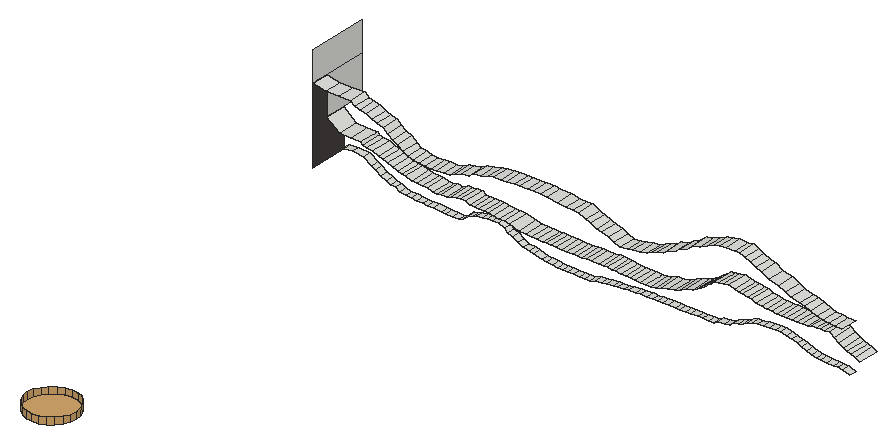
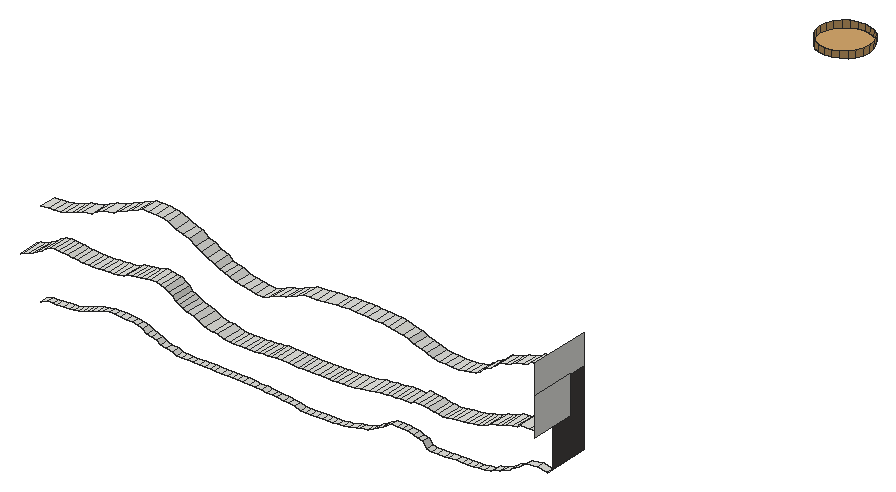
# SketchUp Ruby script. Lengths in inches.
U = 1.inch
M = Sketchup.active_model
def pt(a) = Geom::Point3d.new(a.map { |v| v * U })
def face(e, loops, mat)
  f = e.add_face(loops[0].map { |a| pt(a) })
  loops[1..].each { |l| e.add_face(l.map { |a| pt(a) }).erase! }
  f.material = f.back_material = mat if mat
  f
end
# faces: each face lists its corners as indices into pts; further lists are holes
def faces(e, pts, list, mat = nil) = list.each { |f| face(e, (f[0].is_a?(Array) ? f : [f]).map { |l| l.map { |i| pts[i] } }, mat) }
# xy, xz, yz: faces in a plane at the given z, y or x. An outline is a flat list of corners, or four numbers for a rectangle; further outlines are holes
def ring(l) = l.size == 4 ? [[l[0], l[1]], [l[2], l[1]], [l[2], l[3]], [l[0], l[3]]] : l.each_slice(2).to_a
def flat(e, list, mat, &to3) = list.each { |f| face(e, (f[0].is_a?(Array) ? f : [f]).map { |l| ring(l).map { |u, v| to3.(u, v) } }, mat) }
def xy(e, z, list, mat = nil) = flat(e, list, mat) { |x, y| [x, y, z] }
def xz(e, y, list, mat = nil) = flat(e, list, mat) { |x, z| [x, y, z] }
def yz(e, x, list, mat = nil) = flat(e, list, mat) { |y, z| [x, y, z] }
def lines(e, pts, list) = list.each { |a, b| e.add_line(pt(pts[a]), pt(pts[b])) }
# prism: a flat outline (further loops are holes) pulled along v
def prism(e, loops, v, mat = nil)
  f = face(e, loops, mat); d = Geom::Vector3d.new(v.map { |x| x * U })
  f.pushpull(f.normal.samedirection?(d) ? d.length : -d.length)
end
def box(e, o, s, mat = nil) = prism(e, [[o, [o[0] + s[0], o[1], o[2]], [o[0] + s[0], o[1] + s[1], o[2]], [o[0], o[1] + s[1], o[2]]]], [0, 0, s[2]], mat)
def at(x, y, z, deg = 0) = Geom::Transformation.translation(pt([x, y, z])) * Geom::Transformation.rotation(ORIGIN, Z_AXIS, deg.degrees)
def axes(o, x, y, z) = Geom::Transformation.new([*x, 0, *y, 0, *z, 0, *pt(o).to_a, 1])
def part(name) = M.definitions.add(name)
# library, detail: a bought-in or finely detailed component or shape, given as its bounding box
def library(name, o, s) = part(name).tap { |d| box(d.entities, o, s) }
def detail(e, o, s) = box(e.add_group.entities, o, s)
def put(e, d, t, mat = nil) = e.add_instance(d, t).tap { |i| i.material = mat if mat }
def group(e, t, mat = nil) = e.add_group.tap { |g| g.transformation = t; g.material = mat if mat }.entities
root = M.entities
M.materials.add("[Field Square Tile]").color = [211, 167, 108]
M.materials.add("[Granite Tile]1").color = [68, 65, 63]
xy(root,237.65,[[1160.83,2401.37,1161.52,2402.3],[1161.52,2401.37,1162.14,2402.3]])
xy(root,238.33,[[1169.93,2401.37,1170.48,2402.3],[1170.48,2401.37,1171.16,2402.3]])
xy(root,238.34,[[1171.84,2401.37,1172.77,2402.3],[1172.77,2401.37,1173.26,2402.3],[1173.26,2401.37,1174.02,2402.3],[1174.02,2401.37,1174.65,2402.3],[1174.65,2401.37,1175.4,2402.3],
  [1175.4,2401.37,1176.02,2402.3],[1176.02,2401.37,1176.79,2402.3],[1176.79,2401.37,1177.41,2402.3]])
xy(root,241.52,[[1131.53,2396.68,1131.59,2402.3]])
xy(root,241.68,[[1162.03,2398.8,1162.62,2401.37]])
xy(root,241.75,[[1164.38,2398.8,1165.25,2401.37],[1165.25,2398.8,1165.87,2401.37],[1165.87,2398.8,1166.38,2401.37]])
xy(root,250.6875,[[1151.85,2327.89,1151.06,2328,1150.32,2328.3,1149.68,2328.79,1149.2,2329.43,1148.89,2330.16,1148.79,2330.96,1148.89,2331.75,1149.2,2332.49,1149.68,2333.12,1150.32,2333.61,1151.06,2333.91,1151.85,2334.02,1152.64,2333.91,1153.38,2333.61,1154.01,2333.12,1154.5,2332.49,1154.81,2331.75,1154.91,2330.96,1154.81,2330.16,1154.5,2329.43,1154.01,2328.79,1153.38,2328.3,1152.64,2328]],"[Field Square Tile]")
xz(root,2396.68,[[1131.53,241.52,1131.59,251.5]])
yz(root,1131.59,[[2398.8,246.2,2404.3,250.88],[2396.68,250.88,2404.3,254.5]])
yz(root,1131.59,[[2396.68,241.52,2401.37,241.52,2401.37,246.2,2398.8,246.2,2398.8,250.88,2396.68,250.88]],"[Granite Tile]1")
p = [[1162.14,2401.37,237.65],[1162.14,2402.3,237.65],[1162.81,2402.3,237.89],[1162.81,2401.37,237.89],[1157.47,2401.37,237.76],[1157.47,2402.3,237.76],
  [1158.18,2402.3,237.71],[1158.18,2401.37,237.71],[1158.79,2402.3,237.68],[1158.79,2401.37,237.68],[1159.39,2402.3,237.67],[1159.39,2401.37,237.67],
  [1160.14,2402.3,237.66],[1160.14,2401.37,237.66],[1160.83,2402.3,237.65],[1160.83,2401.37,237.65],[1156.12,2401.37,237.9],[1156.12,2402.3,237.9],
  [1156.78,2402.3,237.82],[1156.78,2401.37,237.82],[1155.18,2401.37,238.21],[1155.18,2402.3,238.21],[1163.57,2402.3,237.94],[1163.57,2401.37,237.94],
  [1164.1875,2402.3,237.98],[1164.1875,2401.37,237.98],[1165.04,2402.3,238.1],[1165.04,2401.37,238.1],[1165.59,2402.3,238.13],[1165.59,2401.37,238.13],
  [1166.35,2402.3,238.15],[1166.35,2401.37,238.15],[1154.71,2401.37,238.31],[1154.71,2402.3,238.31],[1166.98,2402.3,238.26],[1166.98,2401.37,238.26],
  [1153.8,2401.37,238.43],[1153.8,2402.3,238.43],[1167.73,2402.3,238.28],[1167.73,2401.37,238.28],[1168.36,2402.3,238.3],[1168.36,2401.37,238.3],
  [1169.21,2402.3,238.32],[1169.21,2401.37,238.32],[1169.93,2402.3,238.33],[1169.93,2401.37,238.33],[1171.16,2401.37,238.33],[1171.16,2402.3,238.33],
  [1171.84,2402.3,238.34],[1171.84,2401.37,238.34],[1177.41,2401.37,238.34],[1177.41,2402.3,238.34],[1177.92,2402.3,238.59],[1177.92,2401.37,238.59],
  [1153.15,2401.37,238.74],[1153.15,2402.3,238.74],[1193.44,2401.37,238.78],[1193.44,2402.3,238.78],[1194.22,2402.3,238.43],[1194.22,2401.37,238.43],
  [1178.74,2402.3,238.72],[1178.74,2401.37,238.72],[1152.57,2401.37,239.11],[1152.57,2402.3,239.11],[1179.43,2402.3,238.86],[1179.43,2401.37,238.86],
  [1142.78,2401.37,238.92],[1142.78,2402.3,238.92],[1143.82,2402.3,238.82],[1143.82,2401.37,238.82],[1144.33,2402.3,238.8],[1144.33,2401.37,238.8],
  [1145.2,2402.3,238.79],[1145.2,2401.37,238.79],[1145.94,2402.3,238.77],[1145.94,2401.37,238.77],[1146.47,2402.3,238.9375],[1146.47,2401.37,238.9375],
  [1190.72,2401.37,238.875],[1190.72,2402.3,238.875],[1191.47,2402.3,238.83],[1191.47,2401.37,238.83],[1192.23,2402.3,238.8],[1192.23,2401.37,238.8],
  [1192.77,2402.3,238.79],[1192.77,2401.37,238.79],[1140.69,2401.37,238.97],[1140.69,2402.3,238.97],[1141.39,2402.3,238.94],[1141.39,2401.37,238.94],
  [1142.09,2402.3,238.93],[1142.09,2401.37,238.93],[1147.03,2402.3,239.55],[1147.03,2401.37,239.55],[1179.94,2402.3,239.18],[1179.94,2401.37,239.18],
  [1189.57,2401.37,239.04],[1189.57,2402.3,239.04],[1190.15,2402.3,238.94],[1190.15,2401.37,238.94],[1139.32,2401.37,239.09],[1139.32,2402.3,239.09],
  [1140.01,2402.3,239.03],[1140.01,2401.37,239.03],[1188.91,2401.37,239.29],[1188.91,2402.3,239.29],[1138.54,2401.37,239.19],[1138.54,2402.3,239.19],
  [1151.99,2401.37,239.38],[1151.99,2402.3,239.38],[1138.03,2401.37,239.52],[1138.03,2402.3,239.52],[1180.53,2402.3,239.35],[1180.53,2401.37,239.35],
  [1188.33,2401.37,239.53],[1188.33,2402.3,239.53],[1151.53,2401.37,239.71],[1151.53,2402.3,239.71],[1181.09,2402.3,239.52],[1181.09,2401.37,239.52],
  [1137.47,2401.37,239.64],[1137.47,2402.3,239.64],[1181.64,2402.3,239.85],[1181.64,2401.37,239.85],[1187.8,2401.37,239.7],[1187.8,2402.3,239.7],
  [1137.02,2401.37,239.86],[1137.02,2402.3,239.86],[1147.61,2402.3,239.69],[1147.61,2401.37,239.69],[1148.16,2402.3,239.88],[1148.16,2401.37,239.88],
  [1150.83,2401.37,240.11],[1150.83,2402.3,240.11],[1187.11,2401.37,239.92],[1187.11,2402.3,239.92],[1182.28,2402.3,240.03],[1182.28,2401.37,240.03],
  [1136.23,2401.37,240.2],[1136.23,2402.3,240.2],[1148.89,2402.3,239.99],[1148.89,2401.37,239.99],[1186.48,2401.37,240.11],[1186.48,2402.3,240.11],
  [1149.48,2402.3,240.05],[1149.48,2401.37,240.05],[1150.14,2402.3,240.09],[1150.14,2401.37,240.09],[1182.9375,2402.3,240.12],[1182.9375,2401.37,240.12],
  [1183.61,2402.3,240.19],[1183.61,2401.37,240.19],[1185.7,2401.37,240.27],[1185.7,2402.3,240.27],[1135.63,2401.37,240.59],[1135.63,2402.3,240.59],
  [1184.375,2402.3,240.23],[1184.375,2401.37,240.23],[1185.08,2402.3,240.25],[1185.08,2401.37,240.25],[1135.09,2401.37,240.85],[1135.09,2402.3,240.85],
  [1134.07,2401.37,241.55],[1134.07,2402.3,241.55],[1168.01,2398.8,241.57],[1168.01,2401.37,241.57],[1168.55,2401.37,241.53],[1168.55,2398.8,241.53],
  [1169.17,2401.37,241.51],[1169.17,2398.8,241.51],[1169.72,2401.37,241.49],[1169.72,2398.8,241.49],[1170.42,2401.37,241.48],[1170.42,2398.8,241.48],
  [1171.08,2401.37,241.47],[1171.08,2398.8,241.47],[1171.65,2401.37,241.46],[1171.65,2398.8,241.46],[1172.36,2401.37,241.6],[1172.36,2398.8,241.6],
  [1131.59,2401.37,241.52],[1131.59,2402.3,241.52],[1132.8,2402.3,241.69],[1132.8,2401.37,241.69],[1167.4,2398.8,241.66],[1167.4,2401.37,241.66],
  [1173.09,2401.37,241.85],[1173.09,2398.8,241.85],[1158.37,2398.8,241.75],[1158.37,2401.37,241.75],[1158.82,2401.37,241.74],[1158.82,2398.8,241.74],
  [1159.37,2401.37,241.72],[1159.37,2398.8,241.72],[1160,2401.37,241.71],[1160,2398.8,241.71],[1160.63,2401.37,241.7],[1160.63,2398.8,241.7],
  [1161.36,2401.37,241.69],[1161.36,2398.8,241.69],[1162.03,2401.37,241.68],[1162.03,2398.8,241.68],[1162.62,2398.8,241.68],[1162.62,2401.37,241.68],
  [1163.11,2401.37,241.67],[1163.11,2398.8,241.67],[1163.8125,2401.37,241.74],[1163.8125,2398.8,241.74],[1164.38,2401.37,241.75],[1164.38,2398.8,241.75],
  [1166.38,2398.8,241.75],[1166.38,2401.37,241.75],[1166.87,2401.37,241.67],[1166.87,2398.8,241.67],[1156.18,2398.8,241.89],[1156.18,2401.37,241.89],
  [1157,2401.37,241.83],[1157,2398.8,241.83],[1157.6,2401.37,241.78],[1157.6,2398.8,241.78],[1173.76,2401.37,241.91],[1173.76,2398.8,241.91],
  [1155.41,2398.8,241.96],[1155.41,2401.37,241.96],[1174.66,2401.37,242.1],[1174.66,2398.8,242.1],[1154.24,2398.8,242.24],[1154.24,2401.37,242.24],
  [1175.43,2401.37,242.46],[1175.43,2398.8,242.46],[1153.57,2398.8,242.34],[1153.57,2401.37,242.34],[1197.04,2398.8,242.51],[1197.04,2401.37,242.51],
  [1197.55,2401.37,242.21],[1197.55,2398.8,242.21],[1152.91,2398.8,242.38],[1152.91,2401.37,242.38],[1152.25,2398.8,242.48],[1152.25,2401.37,242.48],
  [1144.07,2398.8,242.68],[1144.07,2401.37,242.68],[1144.74,2401.37,242.51],[1144.74,2398.8,242.51],[1145.26,2401.37,242.46],[1145.26,2398.8,242.46],
  [1145.8,2401.37,242.58],[1145.8,2398.8,242.58],[1151.61,2398.8,242.57],[1151.61,2401.37,242.57],[1176.13,2401.37,242.78],[1176.13,2398.8,242.78],
  [1196.45,2398.8,242.68],[1196.45,2401.37,242.68],[1146.43,2401.37,242.57],[1146.43,2398.8,242.57],[1147.06,2401.37,242.81],[1147.06,2398.8,242.81],
  [1148.83,2398.8,242.92],[1148.83,2401.37,242.92],[1149.26,2401.37,242.625],[1149.26,2398.8,242.625],[1149.87,2401.37,242.65],[1149.87,2398.8,242.65],
  [1150.42,2401.37,242.62],[1150.42,2398.8,242.62],[1151.05,2401.37,242.58],[1151.05,2398.8,242.58],[1142.72,2398.8,242.78],[1142.72,2401.37,242.78],
  [1143.53,2401.37,242.73],[1143.53,2398.8,242.73],[1195.95,2398.8,242.875],[1195.95,2401.37,242.875],[1141.42,2398.8,243.06],[1141.42,2401.37,243.06],
  [1142.14,2401.37,242.85],[1142.14,2398.8,242.85],[1147.63,2401.37,242.86],[1147.63,2398.8,242.86],[1176.9,2401.37,242.97],[1176.9,2398.8,242.97],
  [1148.19,2401.37,242.89],[1148.19,2398.8,242.89],[1195.56,2398.8,243.09],[1195.56,2401.37,243.09],[1177.43,2401.37,243.23],[1177.43,2398.8,243.23],
  [1140.35,2398.8,243.3],[1140.35,2401.37,243.3],[1140.9375,2401.37,243.14],[1140.9375,2398.8,243.14],[1194.95,2398.8,243.43],[1194.95,2401.37,243.43],
  [1177.83,2401.37,243.48],[1177.83,2398.8,243.48],[1139.71,2398.8,243.48],[1139.71,2401.37,243.48],[1194.41,2398.8,243.8],[1194.41,2401.37,243.8],
  [1139.19,2398.8,243.79],[1139.19,2401.37,243.79],[1178.35,2401.37,243.72],[1178.35,2398.8,243.72],[1178.6875,2401.37,244.12],[1178.6875,2398.8,244.12],
  [1138.53,2398.8,243.95],[1138.53,2401.37,243.95],[1193.81,2398.8,244.18],[1193.81,2401.37,244.18],[1138.01,2398.8,244.11],[1138.01,2401.37,244.11],
  [1186.63,2398.8,243.99],[1186.63,2401.37,243.99],[1187.35,2401.37,243.95],[1187.35,2398.8,243.95],[1187.85,2401.37,243.93],[1187.85,2398.8,243.93],
  [1188.54,2401.37,243.91],[1188.54,2398.8,243.91],[1189.11,2401.37,243.89],[1189.11,2398.8,243.89],[1189.81,2401.37,243.88],[1189.81,2398.8,243.88],
  [1190.46,2401.37,243.94],[1190.46,2398.8,243.94],[1191.1,2401.37,243.95],[1191.1,2398.8,243.95],[1191.66,2401.37,244.1],[1191.66,2398.8,244.1],
  [1185.45,2398.8,244.11],[1185.45,2401.37,244.11],[1186.01,2401.37,244.04],[1186.01,2398.8,244.04],[1137.34,2398.8,244.41],[1137.34,2401.37,244.41],
  [1179.16,2401.37,244.39],[1179.16,2398.8,244.39],[1184.7,2398.8,244.25],[1184.7,2401.37,244.25],[1192.29,2401.37,244.13],[1192.29,2398.8,244.13],
  [1192.77,2401.37,244.15],[1192.77,2398.8,244.15],[1193.29,2401.37,244.17],[1193.29,2398.8,244.17],[1184.24,2398.8,244.51],[1184.24,2401.37,244.51],
  [1136.58,2398.8,244.54],[1136.58,2401.37,244.54],[1179.64,2401.37,244.73],[1179.64,2398.8,244.73],[1136.02,2398.8,244.61],[1136.02,2401.37,244.61],
  [1183.09,2398.8,244.67],[1183.09,2401.37,244.67],[1183.7,2401.37,244.55],[1183.7,2398.8,244.55],[1135.8,2398.8,244.92],[1135.8,2401.37,244.92],
  [1180.125,2401.37,244.87],[1180.125,2398.8,244.87],[1182.04,2398.8,244.81],[1182.04,2401.37,244.81],[1182.61,2401.37,244.7],[1182.61,2398.8,244.7],
  [1181.39,2398.8,245.01],[1181.39,2401.37,245.01],[1133.16,2398.8,244.96],[1133.16,2401.37,244.96],[1134.55,2401.37,244.9375],[1134.55,2398.8,244.9375],
  [1180.71,2401.37,244.95],[1180.71,2398.8,244.95],[1131.59,2398.8,246.2],[1131.59,2401.37,246.2],[1168.84,2396.68,246.35],[1168.84,2398.8,246.35],
  [1169.61,2398.8,246.05],[1169.61,2396.68,246.05],[1170.51,2398.8,246.13],[1170.51,2396.68,246.13],[1171.22,2398.8,246.29],[1171.22,2396.68,246.29],
  [1172.02,2398.8,246.41],[1172.02,2396.68,246.41],[1168.23,2396.68,246.66],[1168.23,2398.8,246.66],[1172.93,2398.8,246.55],[1172.93,2396.68,246.55],
  [1144.65,2396.68,246.62],[1144.65,2398.8,246.62],[1145.39,2398.8,246.54],[1145.39,2396.68,246.54],[1146.17,2398.8,246.51],[1146.17,2396.68,246.51],
  [1146.95,2398.8,246.58],[1146.95,2396.68,246.58],[1196.14,2396.68,246.59],[1196.14,2398.8,246.59],[1197.03,2398.8,246.55],[1197.03,2396.68,246.55],
  [1143.99,2396.68,246.73],[1143.99,2398.8,246.73],[1147.75,2398.8,246.59],[1147.75,2396.68,246.59],[1148.55,2398.8,246.69],[1148.55,2396.68,246.69],
  [1173.66,2398.8,246.92],[1173.66,2396.68,246.92],[1195.43,2396.68,246.66],[1195.43,2398.8,246.66],[1143.27,2396.68,246.88],[1143.27,2398.8,246.88],
  [1149.26,2398.8,247.03],[1149.26,2396.68,247.03],[1167.375,2396.68,246.94],[1167.375,2398.8,246.94],[1194.64,2396.68,246.75],[1194.64,2398.8,246.75],
  [1193.95,2396.68,246.95],[1193.95,2398.8,246.95],[1142.72,2396.68,247.25],[1142.72,2398.8,247.25],[1166.69,2396.68,247.08],[1166.69,2398.8,247.08],
  [1174.27,2398.8,247.12],[1174.27,2396.68,247.12],[1149.95,2398.8,247.2],[1149.95,2396.68,247.2],[1193.14,2396.68,247.25],[1193.14,2398.8,247.25],
  [1166.01,2396.68,247.46],[1166.01,2398.8,247.46],[1174.95,2398.8,247.31],[1174.95,2396.68,247.31],[1150.92,2398.8,247.39],[1150.92,2396.68,247.39],
  [1192.46,2396.68,247.53],[1192.46,2398.8,247.53],[1142.08,2396.68,247.72],[1142.08,2398.8,247.72],[1175.52,2398.8,247.71],[1175.52,2396.68,247.71],
  [1151.55,2398.8,247.78],[1151.55,2396.68,247.78],[1165.38,2396.68,247.66],[1165.38,2398.8,247.66],[1191.88,2396.68,247.66],[1191.88,2398.8,247.66],
  [1141.43,2396.68,248.07],[1141.43,2398.8,248.07],[1164.54,2396.68,248.08],[1164.54,2398.8,248.08],[1176.45,2398.8,248.03],[1176.45,2396.68,248.03],
  [1190.75,2396.68,247.9],[1190.75,2398.8,247.9],[1152.33,2398.8,247.89],[1152.33,2396.68,247.89],[1153.33,2398.8,248.18],[1153.33,2396.68,248.18],
  [1190.15,2396.68,248.26],[1190.15,2398.8,248.26],[1177.16,2398.8,248.46],[1177.16,2396.68,248.46],[1140.8,2396.68,248.51],[1140.8,2398.8,248.51],
  [1162.92,2396.68,248.15],[1162.92,2398.8,248.15],[1163.74,2398.8,248.11],[1163.74,2396.68,248.11],[1153.97,2398.8,248.29],[1153.97,2396.68,248.29],
  [1161.89,2396.68,248.28],[1161.89,2398.8,248.28],[1154.86,2398.8,248.35],[1154.86,2396.68,248.35],[1160.49,2396.68,248.39],[1160.49,2398.8,248.39],
  [1189.24,2396.68,248.69],[1189.24,2398.8,248.69],[1155.59,2398.8,248.4],[1155.59,2396.68,248.4],[1156.58,2398.8,248.4375],[1156.58,2396.68,248.4375],
  [1157.24,2398.8,248.46],[1157.24,2396.68,248.46],[1159.76,2396.68,248.49],[1159.76,2398.8,248.49],[1140.31,2396.68,249.01],[1140.31,2398.8,249.01],
  [1158.13,2398.8,248.47],[1158.13,2396.68,248.47],[1158.87,2398.8,248.48],[1158.87,2396.68,248.48],[1177.94,2398.8,248.82],[1177.94,2396.68,248.82],
  [1188.02,2396.68,248.95],[1188.02,2398.8,248.95],[1178.66,2398.8,249.37],[1178.66,2396.68,249.37],[1187.13,2396.68,249.46],[1187.13,2398.8,249.46],
  [1139.54,2396.68,249.2],[1139.54,2398.8,249.2],[1138.87,2396.68,249.41],[1138.87,2398.8,249.41],[1138.2,2396.68,249.8],[1138.2,2398.8,249.8],
  [1179.45,2398.8,249.5625],[1179.45,2396.68,249.5625],[1186.37,2396.68,249.68],[1186.37,2398.8,249.68],[1180.35,2398.8,249.9],[1180.35,2396.68,249.9],
  [1185.71,2396.68,250.0625],[1185.71,2398.8,250.0625],[1137.4,2396.68,249.97],[1137.4,2398.8,249.97],[1181.27,2398.8,250.35],[1181.27,2396.68,250.35],
  [1136.79,2396.68,250.15],[1136.79,2398.8,250.15],[1136.26,2396.68,250.55],[1136.26,2398.8,250.55],[1185.02,2396.68,250.32],[1185.02,2398.8,250.32],
  [1181.93,2398.8,250.49],[1181.93,2396.68,250.49],[1184.4,2396.68,250.61],[1184.4,2398.8,250.61],[1131.59,2396.68,250.88],[1131.59,2398.8,250.88],
  [1133.18,2398.8,250.53],[1133.18,2396.68,250.53],[1134.8,2398.8,250.54],[1134.8,2396.68,250.54],[1182.74,2398.8,250.6],[1182.74,2396.68,250.6],
  [1183.76,2398.8,250.58],[1183.76,2396.68,250.58],[1151.85,2327.89,251.5],[1151.06,2328,251.5],[1151.06,2328,250.6875],[1151.85,2327.89,250.6875],
  [1152.64,2328,251.5],[1152.64,2328,250.6875],[1150.32,2328.3,251.5],[1150.32,2328.3,250.6875],[1153.38,2328.3,251.5],[1153.38,2328.3,250.6875],
  [1149.68,2328.79,251.5],[1149.68,2328.79,250.6875],[1154.01,2328.79,251.5],[1154.01,2328.79,250.6875],[1149.2,2329.43,251.5],[1149.2,2329.43,250.6875],
  [1154.5,2329.43,251.5],[1154.5,2329.43,250.6875],[1148.89,2330.16,251.5],[1148.89,2330.16,250.6875],[1154.81,2330.16,251.5],[1154.81,2330.16,250.6875],
  [1148.79,2330.96,251.5],[1148.79,2330.96,250.6875],[1154.91,2330.96,251.5],[1154.91,2330.96,250.6875],[1148.89,2331.75,251.5],[1148.89,2331.75,250.6875],
  [1154.81,2331.75,251.5],[1154.81,2331.75,250.6875],[1149.2,2332.49,251.5],[1149.2,2332.49,250.6875],[1154.5,2332.49,251.5],[1154.5,2332.49,250.6875],
  [1149.68,2333.12,251.5],[1149.68,2333.12,250.6875],[1154.01,2333.12,251.5],[1154.01,2333.12,250.6875],[1150.32,2333.61,251.5],[1150.32,2333.61,250.6875],
  [1153.38,2333.61,251.5],[1153.38,2333.61,250.6875],[1151.06,2333.91,251.5],[1151.06,2333.91,250.6875],[1152.64,2333.91,251.5],[1152.64,2333.91,250.6875],
  [1151.85,2334.02,251.5],[1151.85,2334.02,250.6875]]
faces(root,p,[[0,1,2,3],[4,5,6,7],[7,6,8,9],[9,8,10,11],[11,10,12,13],[13,12,14,15],[16,17,18,19],[19,18,5,4],
  [20,21,17,16],[3,2,22,23],[23,22,24,25],[25,24,26,27],[27,26,28,29],[29,28,30,31],[32,33,21,20],[31,30,34,35],
  [36,37,33,32],[35,34,38,39],[39,38,40,41],[41,40,42,43],[43,42,44,45],[46,47,48,49],[50,51,52,53],[54,55,37,36],
  [56,57,58,59],[53,52,60,61],[62,63,55,54],[61,60,64,65],[66,67,68,69],[69,68,70,71],[71,70,72,73],[73,72,74,75],
  [75,74,76,77],[78,79,80,81],[81,80,82,83],[83,82,84,85],[85,84,57,56],[86,87,88,89],[89,88,90,91],[91,90,67,66],
  [77,76,92,93],[65,64,94,95],[96,97,98,99],[99,98,79,78],[100,101,102,103],[103,102,87,86],[104,105,97,96],[106,107,101,100],
  [108,109,63,62],[110,111,107,106],[95,94,112,113],[114,115,105,104],[116,117,109,108],[113,112,118,119],[120,121,111,110],[119,118,122,123],
  [124,125,115,114],[126,127,121,120],[93,92,128,129],[129,128,130,131],[132,133,117,116],[134,135,125,124],[123,122,136,137],[138,139,127,126],
  [131,130,140,141],[142,143,135,134],[141,140,144,145],[145,144,146,147],[137,136,148,149],[147,146,133,132],[149,148,150,151],[152,153,143,142],
  [154,155,139,138],[151,150,156,157],[157,156,158,159],[159,158,153,152],[160,161,155,154],[162,163,161,160],[164,165,166,167],[167,166,168,169],
  [169,168,170,171],[171,170,172,173],[173,172,174,175],[175,174,176,177],[177,176,178,179],[180,181,182,183],[184,185,165,164],[179,178,186,187],
  [183,182,163,162],[188,189,190,191],[191,190,192,193],[193,192,194,195],[195,194,196,197],[197,196,198,199],[199,198,200,201],[202,203,204,205],
  [205,204,206,207],[207,206,208,209],[210,211,212,213],[213,212,185,184],[214,215,216,217],[217,216,218,219],[219,218,189,188],[187,186,220,221],
  [222,223,215,214],[221,220,224,225],[226,227,223,222],[225,224,228,229],[230,231,227,226],[232,233,234,235],[236,237,231,230],[238,239,237,236],
  [240,241,242,243],[243,242,244,245],[245,244,246,247],[248,249,239,238],[229,228,250,251],[252,253,233,232],[247,246,254,255],[255,254,256,257],
  [258,259,260,261],[261,260,262,263],[263,262,264,265],[265,264,266,267],[267,266,249,248],[268,269,270,271],[271,270,241,240],[272,273,253,252],
  [274,275,276,277],[277,276,269,268],[257,256,278,279],[251,250,280,281],[279,278,282,283],[283,282,259,258],[284,285,273,272],[281,280,286,287],
  [288,289,290,291],[291,290,275,274],[292,293,285,284],[287,286,294,295],[296,297,289,288],[298,299,293,292],[300,301,297,296],[295,294,302,303],
  [303,302,304,305],[306,307,301,300],[308,309,299,298],[310,311,307,306],[312,313,314,315],[315,314,316,317],[317,316,318,319],[319,318,320,321],
  [321,320,322,323],[323,322,324,325],[325,324,326,327],[327,326,328,329],[330,331,332,333],[333,332,313,312],[334,335,311,310],[305,304,336,337],
  [338,339,331,330],[329,328,340,341],[341,340,342,343],[343,342,344,345],[345,344,309,308],[346,347,339,338],[348,349,335,334],[337,336,350,351],
  [352,353,349,348],[354,355,356,357],[357,356,347,346],[358,359,353,352],[351,350,360,361],[362,363,364,365],[365,364,355,354],[366,367,363,362],
  [368,369,370,371],[371,370,359,358],[361,360,372,373],[373,372,367,366],[374,375,369,368],[376,377,378,379],[379,378,380,381],[381,380,382,383],
  [383,382,384,385],[386,387,377,376],[385,384,388,389],[390,391,392,393],[393,392,394,395],[395,394,396,397],[398,399,400,401],[402,403,391,390],
  [397,396,404,405],[405,404,406,407],[389,388,408,409],[410,411,399,398],[412,413,403,402],[407,406,414,415],[416,417,387,386],[418,419,411,410],
  [420,421,419,418],[422,423,413,412],[424,425,417,416],[409,408,426,427],[415,414,428,429],[430,431,421,420],[432,433,425,424],[427,426,434,435],
  [429,428,436,437],[438,439,431,430],[440,441,423,422],[435,434,442,443],[437,436,444,445],[446,447,433,432],[448,449,439,438],[450,451,441,440],
  [452,453,447,446],[443,442,454,455],[456,457,449,448],[445,444,458,459],[459,458,460,461],[462,463,457,456],[455,454,464,465],[466,467,451,450],
  [468,469,470,471],[471,470,453,452],[461,460,472,473],[474,475,469,468],[473,472,476,477],[478,479,475,474],[480,481,463,462],[477,476,482,483],
  [483,482,484,485],[485,484,486,487],[488,489,479,478],[490,491,467,466],[487,486,492,493],[493,492,494,495],[495,494,489,488],[465,464,496,497],
  [498,499,481,480],[497,496,500,501],[502,503,499,498],[504,505,491,490],[506,507,505,504],[508,509,507,506],[501,500,510,511],[512,513,503,502],
  [511,510,514,515],[516,517,513,512],[518,519,509,508],[515,514,520,521],[522,523,519,518],[524,525,523,522],[526,527,517,516],[521,520,528,529],
  [530,531,527,526],[532,533,534,535],[535,534,536,537],[537,536,525,524],[529,528,538,539],[539,538,540,541],[541,540,531,530]])
faces(root,p,[[542,543,544,545],[546,542,545,547],[543,548,549,544],[550,546,547,551],[548,552,553,549],[554,550,551,555],[552,556,557,553],[558,554,555,559],
  [556,560,561,557],[562,558,559,563],[560,564,565,561],[566,562,563,567],[564,568,569,565],[570,566,567,571],[568,572,573,569],[574,570,571,575],
  [572,576,577,573],[578,574,575,579],[576,580,581,577],[582,578,579,583],[580,584,585,581],[586,582,583,587],[584,588,589,585],[588,586,587,589]],"[Field Square Tile]")
